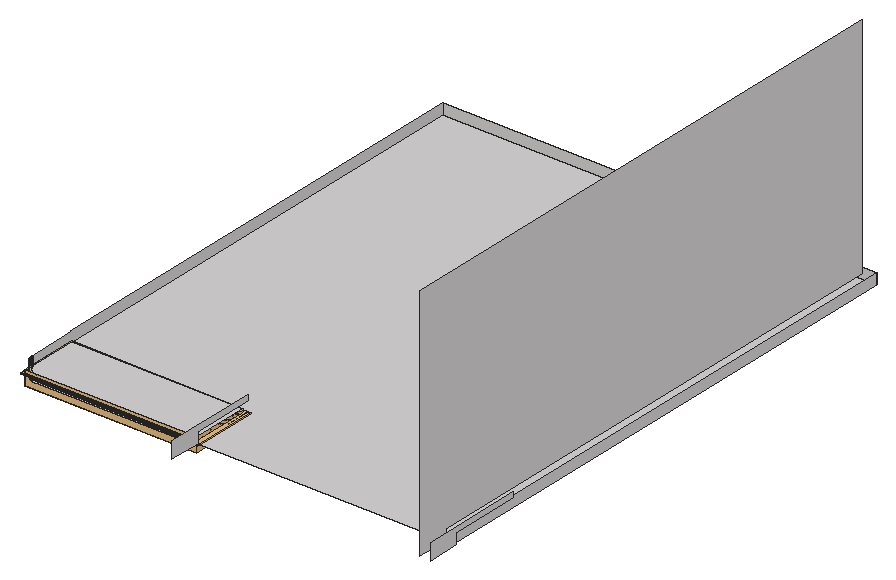
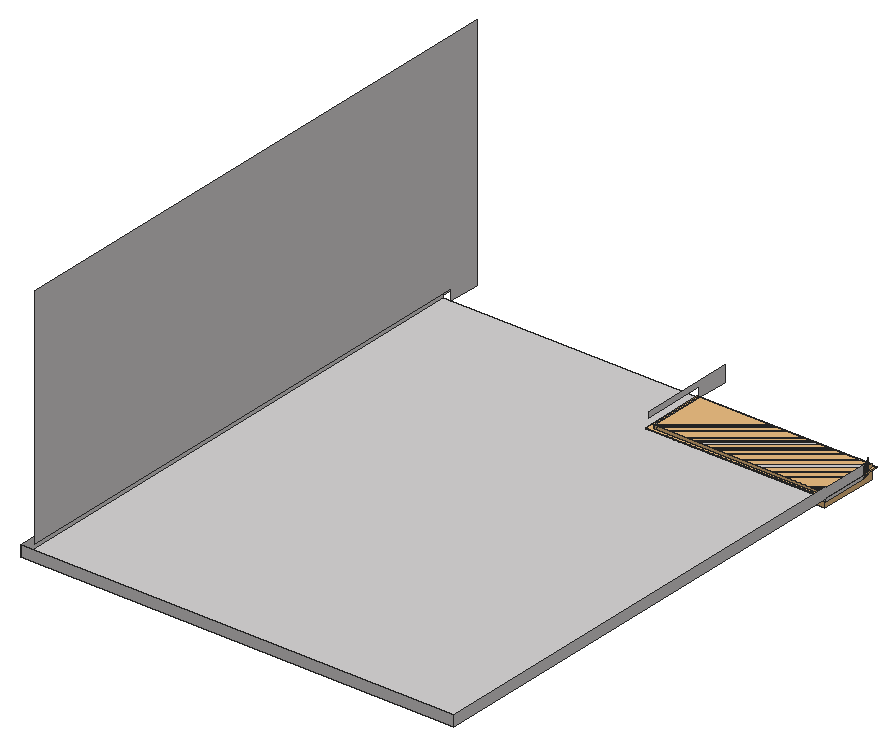
# SketchUp Ruby script. Lengths in inches.
U = 1.inch
M = Sketchup.active_model
def pt(a) = Geom::Point3d.new(a.map { |v| v * U })
def face(e, loops, mat)
  f = e.add_face(loops[0].map { |a| pt(a) })
  loops[1..].each { |l| e.add_face(l.map { |a| pt(a) }).erase! }
  f.material = f.back_material = mat if mat
  f
end
# faces: each face lists its corners as indices into pts; further lists are holes
def faces(e, pts, list, mat = nil) = list.each { |f| face(e, (f[0].is_a?(Array) ? f : [f]).map { |l| l.map { |i| pts[i] } }, mat) }
# xy, xz, yz: faces in a plane at the given z, y or x. An outline is a flat list of corners, or four numbers for a rectangle; further outlines are holes
def ring(l) = l.size == 4 ? [[l[0], l[1]], [l[2], l[1]], [l[2], l[3]], [l[0], l[3]]] : l.each_slice(2).to_a
def flat(e, list, mat, &to3) = list.each { |f| face(e, (f[0].is_a?(Array) ? f : [f]).map { |l| ring(l).map { |u, v| to3.(u, v) } }, mat) }
def xy(e, z, list, mat = nil) = flat(e, list, mat) { |x, y| [x, y, z] }
def xz(e, y, list, mat = nil) = flat(e, list, mat) { |x, z| [x, y, z] }
def yz(e, x, list, mat = nil) = flat(e, list, mat) { |y, z| [x, y, z] }
def lines(e, pts, list) = list.each { |a, b| e.add_line(pt(pts[a]), pt(pts[b])) }
# prism: a flat outline (further loops are holes) pulled along v
def prism(e, loops, v, mat = nil)
  f = face(e, loops, mat); d = Geom::Vector3d.new(v.map { |x| x * U })
  f.pushpull(f.normal.samedirection?(d) ? d.length : -d.length)
end
def box(e, o, s, mat = nil) = prism(e, [[o, [o[0] + s[0], o[1], o[2]], [o[0] + s[0], o[1] + s[1], o[2]], [o[0], o[1] + s[1], o[2]]]], [0, 0, s[2]], mat)
def at(x, y, z, deg = 0) = Geom::Transformation.translation(pt([x, y, z])) * Geom::Transformation.rotation(ORIGIN, Z_AXIS, deg.degrees)
def axes(o, x, y, z) = Geom::Transformation.new([*x, 0, *y, 0, *z, 0, *pt(o).to_a, 1])
def part(name) = M.definitions.add(name)
# library, detail: a bought-in or finely detailed component or shape, given as its bounding box
def library(name, o, s) = part(name).tap { |d| box(d.entities, o, s) }
def detail(e, o, s) = box(e.add_group.entities, o, s)
def put(e, d, t, mat = nil) = e.add_instance(d, t).tap { |i| i.material = mat if mat }
def group(e, t, mat = nil) = e.add_group.tap { |g| g.transformation = t; g.material = mat if mat }.entities
root = M.entities
M.materials.add("Outer Light - 1").color = [251, 216, 141]
M.materials.add("[Quartz Light Brown]").color = [215, 212, 212]
c1 = library("Group\#46",[0,0,-15.9],[195,66,15.9])
c2 = library("Group\#20",[-0.5,-0.5,0],[204,72,1])
xy(root,111,[[[17.76,194,17.53,194.01,17.29,194.01,17.06,194.02,16.82,194.04,16.59,194.06,16.35,194.08,16.12,194.1,15.88,194.125,15.65,194.15,15.42,194.1875,15.18,194.22,14.72,194.3,14.49,194.35,14.26,194.39,14.03,194.44,13.8,194.5,13.57,194.55,13.34,194.61,13.11,194.68,12.89,194.74,12.66,194.81,12.4375,194.88,12.21,194.96,11.99,195.03,11.77,195.11,11.55,195.2,11.33,195.28,10.89,195.46,10.68,195.56,10.46,195.65,10.25,195.75,10.04,195.86,9.83,195.96,9.41,196.18,9.2,196.3,9,196.41,8.6,196.65,8.39,196.78,8.2,196.9,8,197.03,7.8,197.17,7.61,197.3,7.42,197.4375,7.23,197.58,7.04,197.72,6.86,197.86,6.67,198.01,6.49,198.16,6.31,198.3125,6.13,198.47,5.96,198.625,5.78,198.78,5.61,198.94,5.44,199.11,5.27,199.27,5.11,199.44,4.94,199.61,4.78,199.78,4.625,199.96,4.47,200.13,4.3125,200.31,4.16,200.49,4.01,200.67,3.86,200.86,3.72,201.04,3.58,201.23,3.4375,201.42,3.3,201.61,3.17,201.8,3.03,202,2.9,202.2,2.78,202.39,2.65,202.6,2.41,203,2.3,203.2,2.18,203.41,1.96,203.83,1.86,204.04,1.75,204.25,1.65,204.46,1.56,204.68,1.46,204.89,1.28,205.33,1.2,205.55,1.11,205.77,1.03,205.99,0.96,206.21,0.88,206.4375,0.81,206.66,0.74,206.89,0.68,207.11,0.61,207.34,0.55,207.57,0.5,207.8,0.44,208.03,0.39,208.26,0.35,208.49,0.3,208.72,0.22,209.18,0.1875,209.42,0.15,209.65,0.125,209.88,0.1,210.12,0.08,210.35,0.06,210.59,0.04,210.82,0.02,211.06,0.01,211.29,0.01,211.53,0,211.76,0,266,201,266,201,194],[17.8,197,198,197,198,263,3,263,3,211.8,3.01,211.61,3.01,211.41,3.02,211.21,3.03,211.02,3.05,210.82,3.0625,210.63,3.08,210.43,3.1,210.24,3.13,210.04,3.16,209.85,3.18,209.65,3.22,209.46,3.25,209.27,3.29,209.07,3.41,208.5,3.51,208.12,3.5625,207.93,3.62,207.74,3.67,207.55,3.73,207.36,3.8,207.18,3.86,206.99,3.93,206.81,4.07,206.44,4.14,206.26,4.46,205.54,4.55,205.37,4.63,205.19,4.73,205.02,4.82,204.84,4.91,204.67,5.21,204.16,5.3125,204,5.42,203.83,5.53,203.67,5.64,203.5,5.86,203.18,5.98,203.03,6.22,202.71,6.34,202.56,6.47,202.41,6.59,202.26,6.85,201.96,6.99,201.82,7.12,201.67,7.26,201.53,7.39,201.39,7.53,201.26,7.67,201.12,7.82,200.99,7.96,200.85,8.26,200.59,8.41,200.47,8.56,200.34,8.71,200.22,9.03,199.98,9.18,199.86,9.5,199.64,9.67,199.53,9.83,199.42,10,199.3125,10.16,199.21,10.67,198.91,10.84,198.82,11.02,198.73,11.19,198.63,11.37,198.55,11.54,198.46,12.26,198.14,12.44,198.07,12.81,197.93,12.99,197.86,13.18,197.8,13.36,197.73,13.55,197.67,13.74,197.62,13.93,197.5625,14.12,197.51,14.5,197.41,15.07,197.29,15.27,197.25,15.46,197.22,15.65,197.18,15.85,197.16,16.04,197.13,16.24,197.1,16.43,197.08,16.63,197.0625,16.82,197.05,17.02,197.03,17.21,197.02,17.41,197.01,17.61,197.01]]],"[Quartz Light Brown]")
xy(root,114,[[17.76,194,201,194,201,194.5,17.77,194.5,17.54,194.51,17.3125,194.51,17.08,194.52,16.86,194.54,16.625,194.55,16.4,194.57,16.17,194.6,15.94,194.62,15.72,194.65,15.49,194.68,15.26,194.72,15.04,194.75,14.8125,194.79,14.59,194.84,14.36,194.88,14.14,194.93,13.91,194.98,13.03,195.22,12.8125,195.29,12.59,195.36,12.16,195.5,11.94,195.58,11.73,195.66,11.52,195.75,11.3,195.83,10.88,196.01,10.67,196.11,10.47,196.2,10.26,196.3,10.06,196.41,9.85,196.51,9.25,196.84,9.05,196.96,8.86,197.08,8.66,197.2,8.47,197.32,7.71,197.84,6.99,198.4,6.81,198.55,6.63,198.69,6.29,198.99,5.95,199.31,5.79,199.46,5.46,199.79,5.31,199.95,4.99,200.29,4.69,200.63,4.55,200.81,4.4,200.99,3.84,201.71,3.32,202.47,3.2,202.66,3.08,202.86,2.96,203.05,2.84,203.25,2.51,203.85,2.41,204.06,2.3,204.26,2.2,204.47,2.11,204.67,2.01,204.88,1.83,205.3,1.75,205.52,1.66,205.73,1.58,205.94,1.5,206.16,1.36,206.59,1.29,206.8125,1.22,207.03,0.98,207.91,0.93,208.14,0.88,208.36,0.84,208.59,0.79,208.8125,0.75,209.04,0.72,209.26,0.68,209.49,0.65,209.72,0.62,209.94,0.6,210.17,0.57,210.4,0.55,210.625,0.54,210.86,0.52,211.08,0.51,211.3125,0.51,211.54,0.5,211.77,0.5,266,0,266,0,211.76,0.01,211.53,0.01,211.29,0.02,211.06,0.04,210.82,0.06,210.59,0.08,210.35,0.1,210.12,0.125,209.88,0.15,209.65,0.1875,209.42,0.22,209.18,0.3,208.72,0.35,208.49,0.39,208.26,0.44,208.03,0.5,207.8,0.55,207.57,0.61,207.34,0.68,207.11,0.74,206.89,0.81,206.66,0.88,206.4375,0.96,206.21,1.03,205.99,1.11,205.77,1.2,205.55,1.28,205.33,1.46,204.89,1.56,204.68,1.65,204.46,1.75,204.25,1.86,204.04,1.96,203.83,2.18,203.41,2.3,203.2,2.41,203,2.65,202.6,2.78,202.39,2.9,202.2,3.03,202,3.17,201.8,3.3,201.61,3.4375,201.42,3.58,201.23,3.72,201.04,3.86,200.86,4.01,200.67,4.16,200.49,4.3125,200.31,4.47,200.13,4.625,199.96,4.78,199.78,4.94,199.61,5.11,199.44,5.27,199.27,5.44,199.11,5.61,198.94,5.78,198.78,5.96,198.625,6.13,198.47,6.31,198.3125,6.49,198.16,6.67,198.01,6.86,197.86,7.04,197.72,7.23,197.58,7.42,197.4375,7.61,197.3,7.8,197.17,8,197.03,8.2,196.9,8.39,196.78,8.6,196.65,9,196.41,9.2,196.3,9.41,196.18,9.83,195.96,10.04,195.86,10.25,195.75,10.46,195.65,10.68,195.56,10.89,195.46,11.33,195.28,11.55,195.2,11.77,195.11,11.99,195.03,12.21,194.96,12.4375,194.88,12.66,194.81,12.89,194.74,13.11,194.68,13.34,194.61,13.57,194.55,13.8,194.5,14.03,194.44,14.26,194.39,14.49,194.35,14.72,194.3,15.18,194.22,15.42,194.1875,15.65,194.15,15.88,194.125,16.12,194.1,16.35,194.08,16.59,194.06,16.82,194.04,17.06,194.02,17.29,194.01,17.53,194.01],[201,194,201,266,0,266,0,794,492,794,492,194]],"[Quartz Light Brown]")
xy(root,115,[[17.76,194,17.53,194.01,17.29,194.01,17.06,194.02,16.82,194.04,16.59,194.06,16.35,194.08,16.12,194.1,15.88,194.125,15.65,194.15,15.42,194.1875,15.18,194.22,14.72,194.3,14.49,194.35,14.26,194.39,14.03,194.44,13.8,194.5,13.57,194.55,13.34,194.61,13.11,194.68,12.89,194.74,12.66,194.81,12.4375,194.88,12.21,194.96,11.99,195.03,11.77,195.11,11.55,195.2,11.33,195.28,10.89,195.46,10.68,195.56,10.46,195.65,10.25,195.75,10.04,195.86,9.83,195.96,9.41,196.18,9.2,196.3,9,196.41,8.6,196.65,8.39,196.78,8.2,196.9,8,197.03,7.8,197.17,7.61,197.3,7.42,197.4375,7.23,197.58,7.04,197.72,6.86,197.86,6.67,198.01,6.49,198.16,6.31,198.3125,6.13,198.47,5.96,198.625,5.78,198.78,5.61,198.94,5.44,199.11,5.27,199.27,5.11,199.44,4.94,199.61,4.78,199.78,4.625,199.96,4.47,200.13,4.3125,200.31,4.16,200.49,4.01,200.67,3.86,200.86,3.72,201.04,3.58,201.23,3.4375,201.42,3.3,201.61,3.17,201.8,3.03,202,2.9,202.2,2.78,202.39,2.65,202.6,2.41,203,2.3,203.2,2.18,203.41,1.96,203.83,1.86,204.04,1.75,204.25,1.65,204.46,1.56,204.68,1.46,204.89,1.28,205.33,1.2,205.55,1.11,205.77,1.03,205.99,0.96,206.21,0.88,206.4375,0.81,206.66,0.74,206.89,0.68,207.11,0.61,207.34,0.55,207.57,0.5,207.8,0.44,208.03,0.39,208.26,0.35,208.49,0.3,208.72,0.22,209.18,0.1875,209.42,0.15,209.65,0.125,209.88,0.1,210.12,0.08,210.35,0.06,210.59,0.04,210.82,0.02,211.06,0.01,211.29,0.01,211.53,0,211.76,0,266,0.5,266,0.5,211.77,0.51,211.54,0.51,211.3125,0.52,211.08,0.54,210.86,0.55,210.625,0.57,210.4,0.6,210.17,0.62,209.94,0.65,209.72,0.68,209.49,0.72,209.26,0.75,209.04,0.79,208.8125,0.84,208.59,0.88,208.36,0.93,208.14,0.98,207.91,1.22,207.03,1.29,206.8125,1.36,206.59,1.5,206.16,1.58,205.94,1.66,205.73,1.75,205.52,1.83,205.3,2.01,204.88,2.11,204.67,2.2,204.47,2.3,204.26,2.41,204.06,2.51,203.85,2.84,203.25,2.96,203.05,3.08,202.86,3.2,202.66,3.32,202.47,3.84,201.71,4.4,200.99,4.55,200.81,4.69,200.63,4.99,200.29,5.31,199.95,5.46,199.79,5.79,199.46,5.95,199.31,6.29,198.99,6.63,198.69,6.81,198.55,6.99,198.4,7.71,197.84,8.47,197.32,8.66,197.2,8.86,197.08,9.05,196.96,9.25,196.84,9.85,196.51,10.06,196.41,10.26,196.3,10.47,196.2,10.67,196.11,10.88,196.01,11.3,195.83,11.52,195.75,11.73,195.66,11.94,195.58,12.16,195.5,12.59,195.36,12.8125,195.29,13.03,195.22,13.91,194.98,14.14,194.93,14.36,194.88,14.59,194.84,14.8125,194.79,15.04,194.75,15.26,194.72,15.49,194.68,15.72,194.65,15.94,194.62,16.17,194.6,16.4,194.57,16.625,194.55,16.86,194.54,17.08,194.52,17.3125,194.51,17.54,194.51,17.77,194.5,201,194.5,201,194]],"[Quartz Light Brown]")
xy(root,118,[[17.8,197,17.61,197.01,17.41,197.01,17.21,197.02,17.02,197.03,16.82,197.05,16.63,197.0625,16.43,197.08,16.24,197.1,16.04,197.13,15.85,197.16,15.65,197.18,15.46,197.22,15.27,197.25,15.07,197.29,14.5,197.41,14.12,197.51,13.93,197.5625,13.74,197.62,13.55,197.67,13.36,197.73,13.18,197.8,12.99,197.86,12.81,197.93,12.44,198.07,12.26,198.14,11.54,198.46,11.37,198.55,11.19,198.63,11.02,198.73,10.84,198.82,10.67,198.91,10.16,199.21,10,199.3125,9.83,199.42,9.67,199.53,9.5,199.64,9.18,199.86,9.03,199.98,8.71,200.22,8.56,200.34,8.41,200.47,8.26,200.59,7.96,200.85,7.82,200.99,7.67,201.12,7.53,201.26,7.39,201.39,7.26,201.53,7.12,201.67,6.99,201.82,6.85,201.96,6.59,202.26,6.47,202.41,6.34,202.56,6.22,202.71,5.98,203.03,5.86,203.18,5.64,203.5,5.53,203.67,5.42,203.83,5.3125,204,5.21,204.16,4.91,204.67,4.82,204.84,4.73,205.02,4.63,205.19,4.55,205.37,4.46,205.54,4.14,206.26,4.07,206.44,3.93,206.81,3.86,206.99,3.8,207.18,3.73,207.36,3.67,207.55,3.62,207.74,3.5625,207.93,3.51,208.12,3.41,208.5,3.29,209.07,3.25,209.27,3.22,209.46,3.18,209.65,3.16,209.85,3.13,210.04,3.1,210.24,3.08,210.43,3.0625,210.63,3.05,210.82,3.03,211.02,3.02,211.21,3.01,211.41,3.01,211.61,3,211.8,3,263,198,263,198,197]],"[Quartz Light Brown]")
xz(root,263,[[3,111,198,118]],"[Quartz Light Brown]")
xz(root,266,[[0,111,201,114],[0,114,0.5,115]],"[Quartz Light Brown]")
xz(root,794,[[0,114,492,126]],"[Quartz Light Brown]")
yz(root,0,[[211.76,111,212,114],[212,111,266,114],[266,114,266,115,212,115,212,125,266,125,266,126,794,126,794,114],[211.76,115,212,125]],"[Quartz Light Brown]")
yz(root,0.01,[[211.29,111,211.53,114],[211.29,115,211.53,125]],"[Quartz Light Brown]")
yz(root,0.5,[[211.77,114,212,115],[212,114,266,115]],"[Quartz Light Brown]")
yz(root,0.51,[[211.3125,114,211.54,115]],"[Quartz Light Brown]")
yz(root,3,[[211.8,111,212,118],[212,111,263,118]],"[Quartz Light Brown]")
yz(root,3.01,[[211.41,111,211.61,118]],"[Quartz Light Brown]")
yz(root,198,[[197,111,263,118]],"[Quartz Light Brown]")
yz(root,201,[[194,111,266,114],[158,114,158,132,266,132,266,126,194,126,194,114]],"[Quartz Light Brown]")
yz(root,483,[[157.96,114,157.96,384,785,384,785,126,194,126,194,114]],"[Quartz Light Brown]")
yz(root,492,[[194,114,794,126]],"[Quartz Light Brown]")
yz(root,495,[[158,114,194,114,194,126,275,126,275,132,158,132]],"[Quartz Light Brown]")
p = [[8.11,200.72,118],[8.26,200.59,118],[8.26,200.59,111],[8.11,200.72,111],[3.86,200.86,114],[3.86,200.86,111],
  [4.01,200.67,111],[4.01,200.67,114],[7.96,200.85,118],[7.96,200.85,111],[3.72,201.04,114],[3.72,201.04,111],
  [7.82,200.99,118],[7.82,200.99,111],[3.58,201.23,114],[3.58,201.23,111],[7.67,201.12,118],[7.67,201.12,111],
  [7.53,201.26,118],[7.53,201.26,111],[3.4375,201.42,114],[3.4375,201.42,111],[7.39,201.39,118],[7.39,201.39,111],
  [3.3,201.61,114],[3.3,201.61,111],[7.26,201.53,118],[7.26,201.53,111],[7.12,201.67,118],[7.12,201.67,111],
  [3.17,201.8,114],[3.17,201.8,111],[6.99,201.82,118],[6.99,201.82,111],[3.03,202,114],[3.03,202,111],
  [6.85,201.96,118],[6.85,201.96,111],[2.9,202.2,114],[2.9,202.2,111],[6.72,202.11,118],[6.72,202.11,111],
  [6.59,202.26,118],[6.59,202.26,111],[2.78,202.39,114],[2.78,202.39,111],[6.47,202.41,118],[6.47,202.41,111],
  [2.65,202.6,114],[2.65,202.6,111],[6.34,202.56,118],[6.34,202.56,111],[2.53,202.8,114],[2.53,202.8,111],
  [6.22,202.71,118],[6.22,202.71,111],[6.1,202.87,118],[6.1,202.87,111],[2.41,203,114],[2.41,203,111],
  [5.98,203.03,118],[5.98,203.03,111],[2.3,203.2,114],[2.3,203.2,111],[5.86,203.18,118],[5.86,203.18,111],
  [2.18,203.41,114],[2.18,203.41,111],[5.75,203.34,118],[5.75,203.34,111],[5.64,203.5,118],[5.64,203.5,111],
  [2.07,203.62,114],[2.07,203.62,111],[5.53,203.67,118],[5.53,203.67,111],[1.96,203.83,114],[1.96,203.83,111],
  [5.42,203.83,118],[5.42,203.83,111],[1.86,204.04,114],[1.86,204.04,111],[5.3125,204,118],[5.3125,204,111],
  [1.75,204.25,114],[1.75,204.25,111],[5.21,204.16,118],[5.21,204.16,111],[5.11,204.33,118],[5.11,204.33,111],
  [1.65,204.46,114],[1.65,204.46,111],[5.01,204.5,118],[5.01,204.5,111],[1.56,204.68,114],[1.56,204.68,111],
  [4.91,204.67,118],[4.91,204.67,111],[1.46,204.89,114],[1.46,204.89,111],[4.82,204.84,118],[4.82,204.84,111],
  [4.73,205.02,118],[4.73,205.02,111],[1.37,205.11,114],[1.37,205.11,111],[4.63,205.19,118],[4.63,205.19,111],
  [1.28,205.33,114],[1.28,205.33,111],[4.55,205.37,118],[4.55,205.37,111],[1.2,205.55,114],[1.2,205.55,111],
  [4.46,205.54,118],[4.46,205.54,111],[1.11,205.77,114],[1.11,205.77,111],[4.38,205.72,118],[4.38,205.72,111],
  [4.3,205.9,118],[4.3,205.9,111],[1.03,205.99,114],[1.03,205.99,111],[4.22,206.08,118],[4.22,206.08,111],
  [0.96,206.21,114],[0.96,206.21,111],[4.14,206.26,118],[4.14,206.26,111],[0.88,206.4375,114],[0.88,206.4375,111],
  [4.07,206.44,118],[4.07,206.44,111],[0.81,206.66,114],[0.81,206.66,111],[4,206.625,118],[4,206.625,111],
  [3.93,206.81,118],[3.93,206.81,111],[0.74,206.89,114],[0.74,206.89,111],[3.86,206.99,118],[3.86,206.99,111],
  [0.68,207.11,114],[0.68,207.11,111],[3.8,207.18,118],[3.8,207.18,111],[0.61,207.34,114],[0.61,207.34,111],
  [3.73,207.36,118],[3.73,207.36,111],[0.55,207.57,114],[0.55,207.57,111],[3.67,207.55,118],[3.67,207.55,111],
  [0.5,207.8,114],[0.5,207.8,111],[3.62,207.74,118],[3.62,207.74,111],[3.5625,207.93,118],[3.5625,207.93,111],
  [0.44,208.03,114],[0.44,208.03,111],[3.51,208.12,118],[3.51,208.12,111],[0.39,208.26,114],[0.39,208.26,111],
  [3.46,208.31,118],[3.46,208.31,111],[0.35,208.49,114],[0.35,208.49,111],[3.41,208.5,118],[3.41,208.5,111],
  [0.3,208.72,114],[0.3,208.72,111],[3.37,208.69,118],[3.37,208.69,111],[0.26,208.95,114],[0.26,208.95,111],
  [3.33,208.88,118],[3.33,208.88,111],[3.29,209.07,118],[3.29,209.07,111],[0.22,209.18,114],[0.22,209.18,111],
  [3.25,209.27,118],[3.25,209.27,111],[0.1875,209.42,114],[0.1875,209.42,111],[3.22,209.46,118],[3.22,209.46,111],
  [0.15,209.65,114],[0.15,209.65,111],[3.18,209.65,118],[3.18,209.65,111],[0.125,209.88,114],[0.125,209.88,111],
  [3.16,209.85,118],[3.16,209.85,111],[3.13,210.04,118],[3.13,210.04,111],[0.1,210.12,114],[0.1,210.12,111],
  [3.1,210.24,118],[3.1,210.24,111],[0.08,210.35,114],[0.08,210.35,111],[3.08,210.43,118],[3.08,210.43,111],
  [0.06,210.59,114],[0.06,210.59,111],[3.0625,210.63,118],[3.0625,210.63,111],[0.04,210.82,114],[0.04,210.82,111],
  [3.05,210.82,118],[3.05,210.82,111],[0.02,211.06,114],[0.02,211.06,111],[3.03,211.02,118],[3.03,211.02,111],
  [3.02,211.21,118],[3.02,211.21,111],[0.01,211.29,114],[0.01,211.29,111],[3.01,211.41,118],[3.01,211.41,111],
  [0,211.76,114],[0,211.76,111],[0.01,211.53,111],[0.01,211.53,114],[3,211.8,118],[3.01,211.61,118],
  [3.01,211.61,111],[3,211.8,111],[4.55,200.81,115],[4.55,200.81,114],[4.69,200.63,114],[4.69,200.63,115],
  [4.4,200.99,115],[4.4,200.99,114],[4.26,201.17,115],[4.26,201.17,114],[4.12,201.35,115],[4.12,201.35,114],
  [3.98,201.53,115],[3.98,201.53,114],[3.84,201.71,115],[3.84,201.71,114],[3.71,201.9,115],[3.71,201.9,114],
  [3.58,202.09,115],[3.58,202.09,114],[3.45,202.28,115],[3.45,202.28,114],[3.32,202.47,115],[3.32,202.47,114],
  [3.2,202.66,115],[3.2,202.66,114],[3.08,202.86,115],[3.08,202.86,114],[2.96,203.05,115],[2.96,203.05,114],
  [2.84,203.25,115],[2.84,203.25,114],[2.73,203.45,115],[2.73,203.45,114],[2.62,203.65,115],[2.62,203.65,114],
  [2.51,203.85,115],[2.51,203.85,114],[2.41,204.06,115],[2.41,204.06,114],[2.3,204.26,115],[2.3,204.26,114],
  [2.2,204.47,115],[2.2,204.47,114],[2.11,204.67,115],[2.11,204.67,114],[2.01,204.88,115],[2.01,204.88,114],
  [1.92,205.09,115],[1.92,205.09,114],[1.83,205.3,115],[1.83,205.3,114],[1.75,205.52,115],[1.75,205.52,114],
  [1.66,205.73,115],[1.66,205.73,114],[1.58,205.94,115],[1.58,205.94,114],[1.5,206.16,115],[1.5,206.16,114],
  [1.43,206.375,115],[1.43,206.375,114],[1.36,206.59,115],[1.36,206.59,114],[1.29,206.8125,115],[1.29,206.8125,114],
  [1.22,207.03,115],[1.22,207.03,114],[1.16,207.25,115],[1.16,207.25,114],[1.1,207.47,115],[1.1,207.47,114],
  [1.04,207.69,115],[1.04,207.69,114],[0.98,207.91,115],[0.98,207.91,114],[0.93,208.14,115],[0.93,208.14,114],
  [0.88,208.36,115],[0.88,208.36,114],[0.84,208.59,115],[0.84,208.59,114],[0.79,208.8125,115],[0.79,208.8125,114],
  [0.75,209.04,115],[0.75,209.04,114],[0.72,209.26,115],[0.72,209.26,114],[0.68,209.49,115],[0.68,209.49,114],
  [0.65,209.72,115],[0.65,209.72,114],[0.62,209.94,115],[0.62,209.94,114],[0.6,210.17,115],[0.6,210.17,114],
  [0.57,210.4,115],[0.57,210.4,114],[0.55,210.625,115],[0.55,210.625,114],[0.54,210.86,115],[0.54,210.86,114],
  [0.52,211.08,115],[0.52,211.08,114],[0.51,211.3125,115],[0.51,211.3125,114],[0.5,211.77,115],[0.5,211.77,114],
  [0.51,211.54,114],[0.51,211.54,115],[4.01,200.67,125],[4.01,200.67,115],[4.16,200.49,115],[4.16,200.49,125],
  [3.86,200.86,125],[3.86,200.86,115],[3.72,201.04,125],[3.72,201.04,115],[3.58,201.23,125],[3.58,201.23,115],
  [3.4375,201.42,125],[3.4375,201.42,115],[3.3,201.61,125],[3.3,201.61,115],[3.17,201.8,125],[3.17,201.8,115],
  [3.03,202,125],[3.03,202,115],[2.9,202.2,125],[2.9,202.2,115],[2.78,202.39,125],[2.78,202.39,115],
  [2.65,202.6,125],[2.65,202.6,115],[2.53,202.8,125],[2.53,202.8,115],[2.41,203,125],[2.41,203,115],
  [2.3,203.2,125],[2.3,203.2,115],[2.18,203.41,125],[2.18,203.41,115],[2.07,203.62,125],[2.07,203.62,115],
  [1.96,203.83,125],[1.96,203.83,115],[1.86,204.04,125],[1.86,204.04,115],[1.75,204.25,125],[1.75,204.25,115],
  [1.65,204.46,125],[1.65,204.46,115],[1.56,204.68,125],[1.56,204.68,115],[1.46,204.89,125],[1.46,204.89,115],
  [1.37,205.11,125],[1.37,205.11,115],[1.28,205.33,125],[1.28,205.33,115],[1.2,205.55,125],[1.2,205.55,115],
  [1.11,205.77,125],[1.11,205.77,115],[1.03,205.99,125],[1.03,205.99,115],[0.96,206.21,125],[0.96,206.21,115],
  [0.88,206.4375,125],[0.88,206.4375,115],[0.81,206.66,125],[0.81,206.66,115],[0.74,206.89,125],[0.74,206.89,115],
  [0.68,207.11,125],[0.68,207.11,115],[0.61,207.34,125],[0.61,207.34,115],[0.55,207.57,125],[0.55,207.57,115],
  [0.5,207.8,125],[0.5,207.8,115],[0.44,208.03,125],[0.44,208.03,115],[0.39,208.26,125],[0.39,208.26,115],
  [0.35,208.49,125],[0.35,208.49,115],[0.3,208.72,125],[0.3,208.72,115],[0.26,208.95,125],[0.26,208.95,115],
  [0.22,209.18,125],[0.22,209.18,115],[0.1875,209.42,125],[0.1875,209.42,115],[0.15,209.65,125],[0.15,209.65,115],
  [0.125,209.88,125],[0.125,209.88,115],[0.1,210.12,125],[0.1,210.12,115],[0.08,210.35,125],[0.08,210.35,115],
  [0.06,210.59,125],[0.06,210.59,115],[0.04,210.82,125],[0.04,210.82,115],[0.02,211.06,125],[0.02,211.06,115],
  [0.01,211.29,125],[0.01,211.29,115],[0,211.76,125],[0,211.76,115],[0.01,211.53,115],[0.01,211.53,125]]
faces(root,p,[[0,1,2,3],[4,5,6,7],[8,0,3,9],[10,11,5,4],[12,8,9,13],[14,15,11,10],[16,12,13,17],[18,16,17,19],
  [20,21,15,14],[22,18,19,23],[24,25,21,20],[26,22,23,27],[28,26,27,29],[30,31,25,24],[32,28,29,33],[34,35,31,30],
  [36,32,33,37],[38,39,35,34],[40,36,37,41],[42,40,41,43],[44,45,39,38],[46,42,43,47],[48,49,45,44],[50,46,47,51],
  [52,53,49,48],[54,50,51,55],[56,54,55,57],[58,59,53,52],[60,56,57,61],[62,63,59,58],[64,60,61,65],[66,67,63,62],
  [68,64,65,69],[70,68,69,71],[72,73,67,66],[74,70,71,75],[76,77,73,72],[78,74,75,79],[80,81,77,76],[82,78,79,83],
  [84,85,81,80],[86,82,83,87],[88,86,87,89],[90,91,85,84],[92,88,89,93],[94,95,91,90],[96,92,93,97],[98,99,95,94],
  [100,96,97,101],[102,100,101,103],[104,105,99,98],[106,102,103,107],[108,109,105,104],[110,106,107,111],[112,113,109,108],[114,110,111,115],
  [116,117,113,112],[118,114,115,119],[120,118,119,121],[122,123,117,116],[124,120,121,125],[126,127,123,122],[128,124,125,129],[130,131,127,126],
  [132,128,129,133],[134,135,131,130],[136,132,133,137],[138,136,137,139],[140,141,135,134],[142,138,139,143],[144,145,141,140],[146,142,143,147],
  [148,149,145,144],[150,146,147,151],[152,153,149,148],[154,150,151,155],[156,157,153,152],[158,154,155,159],[160,158,159,161],[162,163,157,156],
  [164,160,161,165],[166,167,163,162],[168,164,165,169],[170,171,167,166],[172,168,169,173],[174,175,171,170],[176,172,173,177],[178,179,175,174],
  [180,176,177,181],[182,180,181,183],[184,185,179,178],[186,182,183,187],[188,189,185,184],[190,186,187,191],[192,193,189,188],[194,190,191,195],
  [196,197,193,192],[198,194,195,199],[200,198,199,201],[202,203,197,196],[204,200,201,205],[206,207,203,202],[208,204,205,209],[210,211,207,206],
  [212,208,209,213],[214,215,211,210],[216,212,213,217],[218,219,215,214],[220,216,217,221],[222,220,221,223],[224,225,219,218],[226,222,223,227],
  [228,229,230,231],[232,233,234,235],[236,237,238,239],[240,241,237,236],[242,243,241,240],[244,245,243,242],[246,247,245,244],[248,249,247,246],
  [250,251,249,248],[252,253,251,250],[254,255,253,252],[256,257,255,254],[258,259,257,256],[260,261,259,258],[262,263,261,260],[264,265,263,262],
  [266,267,265,264],[268,269,267,266],[270,271,269,268],[272,273,271,270],[274,275,273,272],[276,277,275,274],[278,279,277,276],[280,281,279,278],
  [282,283,281,280],[284,285,283,282],[286,287,285,284],[288,289,287,286],[290,291,289,288],[292,293,291,290],[294,295,293,292],[296,297,295,294],
  [298,299,297,296],[300,301,299,298],[302,303,301,300],[304,305,303,302],[306,307,305,304],[308,309,307,306],[310,311,309,308],[312,313,311,310],
  [314,315,313,312],[316,317,315,314],[318,319,317,316],[320,321,319,318],[322,323,321,320],[324,325,323,322],[326,327,325,324],[328,329,327,326],
  [330,331,329,328],[332,333,331,330],[334,335,333,332],[336,337,335,334],[338,339,337,336],[340,341,342,343],[344,345,346,347],[348,349,345,344],
  [350,351,349,348],[352,353,351,350],[354,355,353,352],[356,357,355,354],[358,359,357,356],[360,361,359,358],[362,363,361,360],[364,365,363,362],
  [366,367,365,364],[368,369,367,366],[370,371,369,368],[372,373,371,370],[374,375,373,372],[376,377,375,374],[378,379,377,376],[380,381,379,378],
  [382,383,381,380],[384,385,383,382],[386,387,385,384],[388,389,387,386],[390,391,389,388],[392,393,391,390],[394,395,393,392],[396,397,395,394],
  [398,399,397,396],[400,401,399,398],[402,403,401,400],[404,405,403,402],[406,407,405,404],[408,409,407,406],[410,411,409,408],[412,413,411,410],
  [414,415,413,412],[416,417,415,414],[418,419,417,416],[420,421,419,418],[422,423,421,420],[424,425,423,422],[426,427,425,424],[428,429,427,426],
  [430,431,429,428],[432,433,431,430],[434,435,433,432],[436,437,435,434],[438,439,437,436],[440,441,439,438],[442,443,441,440],[444,445,443,442],
  [446,447,448,449]],"[Quartz Light Brown]")
put(root,c1,at(3,197,118),"[Quartz Light Brown]")
put(root,c2,at(0.5,194.5,114),"Outer Light - 1")
